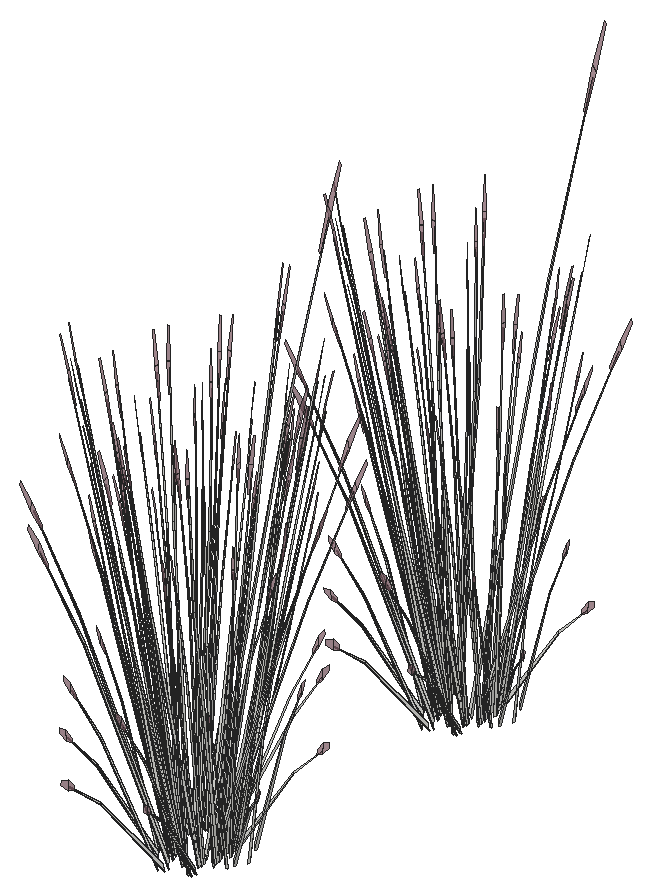
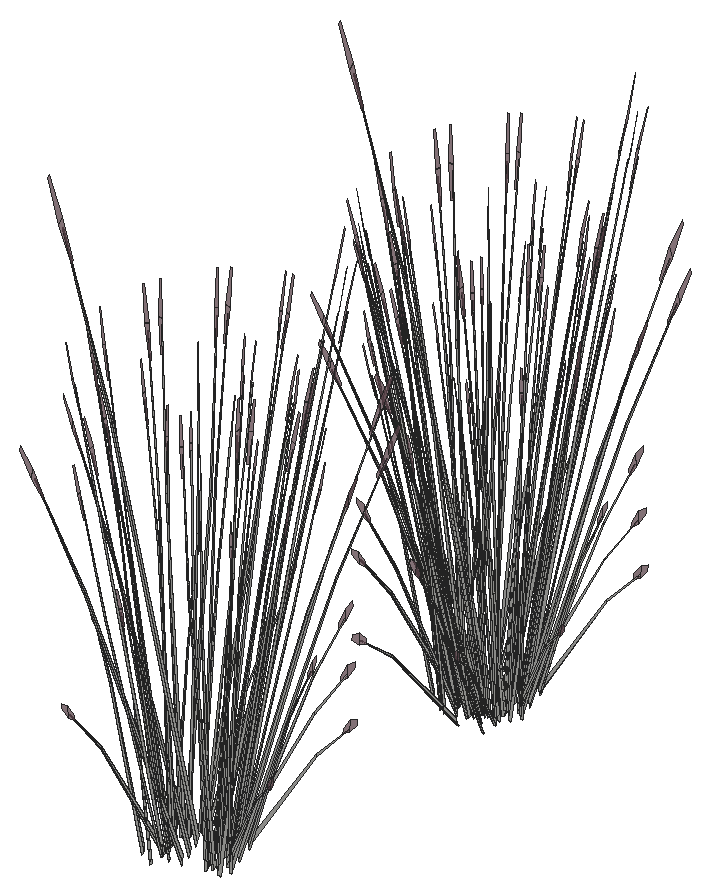
# SketchUp Ruby script. Lengths in inches.
U = 1.inch
M = Sketchup.active_model
def pt(a) = Geom::Point3d.new(a.map { |v| v * U })
def face(e, loops, mat)
  f = e.add_face(loops[0].map { |a| pt(a) })
  loops[1..].each { |l| e.add_face(l.map { |a| pt(a) }).erase! }
  f.material = f.back_material = mat if mat
  f
end
# faces: each face lists its corners as indices into pts; further lists are holes
def faces(e, pts, list, mat = nil) = list.each { |f| face(e, (f[0].is_a?(Array) ? f : [f]).map { |l| l.map { |i| pts[i] } }, mat) }
# xy, xz, yz: faces in a plane at the given z, y or x. An outline is a flat list of corners, or four numbers for a rectangle; further outlines are holes
def ring(l) = l.size == 4 ? [[l[0], l[1]], [l[2], l[1]], [l[2], l[3]], [l[0], l[3]]] : l.each_slice(2).to_a
def flat(e, list, mat, &to3) = list.each { |f| face(e, (f[0].is_a?(Array) ? f : [f]).map { |l| ring(l).map { |u, v| to3.(u, v) } }, mat) }
def xy(e, z, list, mat = nil) = flat(e, list, mat) { |x, y| [x, y, z] }
def xz(e, y, list, mat = nil) = flat(e, list, mat) { |x, z| [x, y, z] }
def yz(e, x, list, mat = nil) = flat(e, list, mat) { |y, z| [x, y, z] }
def lines(e, pts, list) = list.each { |a, b| e.add_line(pt(pts[a]), pt(pts[b])) }
# prism: a flat outline (further loops are holes) pulled along v
def prism(e, loops, v, mat = nil)
  f = face(e, loops, mat); d = Geom::Vector3d.new(v.map { |x| x * U })
  f.pushpull(f.normal.samedirection?(d) ? d.length : -d.length)
end
def box(e, o, s, mat = nil) = prism(e, [[o, [o[0] + s[0], o[1], o[2]], [o[0] + s[0], o[1] + s[1], o[2]], [o[0], o[1] + s[1], o[2]]]], [0, 0, s[2]], mat)
def at(x, y, z, deg = 0) = Geom::Transformation.translation(pt([x, y, z])) * Geom::Transformation.rotation(ORIGIN, Z_AXIS, deg.degrees)
def axes(o, x, y, z) = Geom::Transformation.new([*x, 0, *y, 0, *z, 0, *pt(o).to_a, 1])
def part(name) = M.definitions.add(name)
# library, detail: a bought-in or finely detailed component or shape, given as its bounding box
def library(name, o, s) = part(name).tap { |d| box(d.entities, o, s) }
def detail(e, o, s) = box(e.add_group.entities, o, s)
def put(e, d, t, mat = nil) = e.add_instance(d, t).tap { |i| i.material = mat if mat }
def group(e, t, mat = nil) = e.add_group.tap { |g| g.transformation = t; g.material = mat if mat }.entities
root = M.entities
M.materials.add("LightPink_Translucent").color = [144, 107, 117]
M.materials["LightPink_Translucent"].alpha = 0.75
c1 = part("blade")
p = [[2.15,0.21,22],[0,0.17,0],[0.09,0.45,0],[2.18,0.31,22],[2.29,0.31,22],[0.38,0.45,0],
  [2.48,0.24,33],[2.49,0.24,33],[2.48,0.22,33]]
faces(c1.entities,p,[[0,1,2,3],[4,5,2,3],[6,3,4,7],[8,0,3,6]])
c2 = part("seeds")
p = [[0.3,-0.1,1.38],[-0.01,-0.03,1.59],[-0.01,-0.03,0.03],[0.14,-0.07,-0.07],[0.29,-0.03,3],[0.15,0.01,3.11]]
faces(c2.entities,p,[[0,1,2,3],[1,0,4,5]],"LightPink_Translucent")
c3 = part("blade with seeds")
put(c3.entities,c1,at(0,0,0))
put(c3.entities,c2,axes([2.4,0.25,30.99],[1.5799,-0.05474,1.17369],[-0.12525,1.92788,0.29478],[-0.07173,-0.02425,1.56792]))
put(root,c3,axes([430.05,19.08,1.33],[0.08601,0.17716,1.47384],[-0.39746,0.14915,0.11917],[-0.08983,-0.27813,0.63005]))
put(root,c3,axes([430.7,17.9,2.05],[-0.05755,-0.07737,1.50452],[-0.38409,0.04905,-0.23794],[-0.0613,-0.18505,0.12066]))
put(root,c3,axes([432.43,18.85,2.05],[-0.00363,-0.10982,1.50452],[-0.30678,-0.3174,-0.23794],[0.04743,-0.1924,0.12066]))
put(root,c3,axes([431.39,19.39,1.33],[-0.07006,0.18966,1.47384],[-0.29392,-0.3925,0.11917],[0.13259,-0.24463,0.63005]))
put(root,c3,axes([432.35,18.46,2.05],[-0.03821,0.04215,1.5255],[-0.37441,-0.1422,-0.14414],[-0.01355,-0.18393,0.26996]))
put(root,c3,axes([430.31,17.65,2.05],[-0.00702,0.06614,1.5255],[-0.34622,0.24004,-0.14414],[-0.10188,-0.1227,0.26996]))
put(root,c3,axes([430.23,18.82,2.38],[0.41917,-0.14183,0.46236],[0.07275,0.55635,0.38124],[-0.09858,-0.16397,0.95674]))
put(root,c3,axes([431.18,18.93,2.07],[0.37078,0.14426,0.41282],[-0.12679,0.47426,0.34039],[-0.02228,-0.18651,0.85423]))
put(root,c3,axes([431.29,19.1,2.33],[-0.36822,0.25691,-0.10458],[-0.18095,-0.45596,-0.58045],[-0.04858,-0.19215,0.88199]))
put(root,c3,axes([432.05,19.67,2.33],[-0.41355,-0.02734,-0.10458],[0.0113,-0.51765,-0.58045],[0.02873,-0.19937,0.88199]))
put(root,c3,axes([431.28,18.89,2.07],[0.27727,-0.18753,0.0553],[0.13571,0.34197,0.43534],[-0.02678,-0.15075,0.66383]))
put(root,c3,axes([430.33,18.94,2.07],[0.17102,-0.35053,0.0553],[0.24354,0.20408,0.43534],[-0.07874,-0.11238,0.66383]))
put(root,c3,axes([429.47,19.63,1.33],[0.13977,0.09507,1.47384],[-0.28925,0.39884,0.11917],[-0.18028,-0.17992,0.63005]))
put(root,c3,axes([431.18,19.28,2.34],[-0.11344,0.42434,0.30456],[-0.33096,-0.12377,-0.39319],[-0.03035,-0.17085,0.75234]))
put(root,c3,axes([432.02,19.46,2.07],[0.26795,0.37649,0.41282],[-0.28456,0.3247,0.34039],[0.04943,-0.17664,0.85423]))
put(root,c3,axes([430.41,18.91,2.67],[-0.25113,0.52899,-0.11713],[-0.36369,-0.30476,-0.65011],[-0.12642,-0.14945,0.98783]))
put(root,c3,axes([432.12,19.49,2.07],[0.30922,0.02571,0.0553],[-0.00848,0.38824,0.43534],[0.03236,-0.14872,0.66383]))
put(root,c3,axes([431.89,19.75,2.34],[-0.2546,0.29052,0.30456],[-0.24101,-0.33173,-0.39319],[0.03667,-0.16855,0.75234]))
put(root,c3,axes([429.44,18.76,2.05],[-0.08096,-0.00389,1.50452],[-0.25776,0.38949,-0.23794],[-0.13753,-0.07958,0.12066]))
put(root,c3,axes([432.5,20.69,2.33],[-0.34807,-0.30426,-0.10458],[0.20053,-0.44063,-0.58045],[0.09834,-0.15317,0.88199]))
put(root,c3,axes([430.38,19.35,2.34],[0.05812,0.44446,0.30456],[-0.33222,0.11736,-0.39319],[-0.08923,-0.12737,0.75234]))
put(root,c3,axes([429.38,19.64,2.38],[0.31075,-0.40722,0.46236],[0.268,0.43246,0.38124],[-0.14579,-0.07512,0.95674]))
put(root,c3,axes([433.36,20.5625,2.05],[-0.04915,-0.00419,1.5255],[-0.20409,-0.44904,-0.14414],[0.08196,-0.14765,0.26996]))
put(root,c3,axes([429.53,19.63,2.07],[0.01895,-0.4196,0.0553],[0.28611,0.0115,0.43534],[-0.1096,-0.04391,0.66383]))
put(root,c3,axes([432.33,20.65,2.34],[-0.32754,0.07886,0.30456],[-0.08649,-0.45081,-0.39319],[0.09386,-0.12109,0.75234]))
put(root,c3,axes([432.63,20.58,2.07],[0.25832,0.23207,0.0553],[-0.1504,0.33047,0.43534],[0.08282,-0.10684,0.66383]))
put(root,c3,axes([432.56,20.48,2.07],[0.09332,0.50785,0.41282],[-0.36608,0.08814,0.34039],[0.10789,-0.11944,0.85423]))
put(root,c3,axes([433.54,21.1,2.05],[0.05222,-0.08405,1.50452],[-0.06683,-0.51557,-0.23794],[0.13101,-0.09775,0.12066]))
put(root,c3,axes([429.13,19.09,2.05],[0.0279,0.05507,1.5255],[-0.13448,0.49501,-0.14414],[-0.1362,0.00358,0.26996]))
put(root,c3,axes([429.72,19.95,2.34],[0.2141,0.34548,0.30456],[-0.24447,0.32704,-0.39319],[-0.12421,-0.04976,0.75234]))
put(root,c3,axes([429.66,19.73,2.33],[-0.02015,0.56117,-0.10458],[-0.38148,-0.01534,-0.58045],[-0.14692,-0.03898,0.88199]))
put(root,c3,axes([432.52,21.88,2.33],[-0.18933,-0.49965,-0.10458],[0.33602,-0.24554,-0.58045],[0.1416,-0.06592,0.88199]))
put(root,c3,axes([429.18,20.5,1.33],[0.15608,-0.0125,1.47384],[-0.10354,0.54165,0.11917],[-0.22242,-0.0335,0.63005]))
put(root,c3,axes([432.38,21.73,2.34],[-0.31272,-0.15393,0.30456],[0.09121,-0.44909,-0.39319],[0.1259,-0.04118,0.75234]))
put(root,c3,axes([429.11,20.91,2.07],[0.10631,-0.50312,0.41282],[0.34951,0.17204,0.34039],[-0.13745,0.03024,0.85423]))
put(root,c3,axes([429.08,20.78,2.07],[-0.1382,-0.37624,0.0553],[0.25202,-0.18416,0.43534],[-0.11109,0.03633,0.66383]))
put(root,c3,axes([431.86,21.125,1.33],[-0.15608,0.0125,1.47384],[0.10354,-0.54165,0.11917],[0.22242,0.0335,0.63005]))
put(root,c3,axes([432.67,21.87,2.07],[0.1382,0.37624,0.0553],[-0.25202,0.18416,0.43534],[0.11109,-0.03633,0.66383]))
put(root,c3,axes([432.64,21.74,2.07],[-0.10631,0.50312,0.41282],[-0.34951,-0.17204,0.34039],[0.13745,-0.03024,0.85423]))
put(root,c3,axes([429.37,20.92,2.34],[0.31272,0.15393,0.30456],[-0.09121,0.44909,-0.39319],[-0.1259,0.04118,0.75234]))
put(root,c3,axes([433.27,23.37,2.05],[-0.03403,-0.04831,1.5255],[0.07443,-0.51782,-0.14414],[0.13402,-0.03308,0.26996]))
put(root,c3,axes([428.84,21.26,2.05],[-0.06145,0.07164,1.50452],[0.00523,0.52344,-0.23794],[-0.14085,0.06807,0.12066]))
put(root,c3,axes([429.24,20.77,2.33],[0.18933,0.49965,-0.10458],[-0.33602,0.24554,-0.58045],[-0.1416,0.06592,0.88199]))
put(root,c3,axes([432.97,22.93,1.38],[-0.07202,-0.46385,-0.03003],[0.3404,-0.10664,-0.13615],[0.07108,0.02941,0.44908]))
put(root,c3,axes([432.09,22.92,2.33],[0.02015,-0.56117,-0.10458],[0.38148,0.01534,-0.58045],[0.14692,0.03898,0.88199]))
put(root,c3,axes([432.03,22.7,2.34],[-0.2141,-0.34548,0.30456],[0.24447,-0.32704,-0.39319],[0.12421,0.04976,0.75234]))
put(root,c3,axes([432.42,22.58,2.05],[0.08072,-0.00933,1.50452],[0.22141,-0.42869,-0.23794],[0.14358,0.05659,0.12066]))
put(root,c3,axes([429.2,22.16,2.07],[-0.09332,-0.50785,0.41282],[0.36608,-0.08814,0.34039],[-0.10789,0.11944,0.85423]))
put(root,c3,axes([429.125,22.07,2.07],[-0.25832,-0.23207,0.0553],[0.1504,-0.33047,0.43534],[-0.08282,0.10684,0.66383]))
put(root,c3,axes([429.24,21.45,1.33],[0.13056,-0.11672,1.47384],[0.10992,0.53933,0.11917],[-0.20497,0.12189,0.63005]))
put(root,c3,axes([429.42,21.99,2.34],[0.32754,-0.07886,0.30456],[0.08649,0.45081,-0.39319],[-0.09386,0.12109,0.75234]))
put(root,c3,axes([428.16,21.79,2.05],[0.04802,0.0148,1.5255],[0.14856,0.48754,-0.14414],[-0.0983,0.12796,0.26996]))
put(root,c3,axes([432.23,23.01,2.07],[-0.01895,0.4196,0.0553],[-0.28611,-0.0115,0.43534],[0.1096,0.04391,0.66383]))
put(root,c3,axes([432.25,22.88,2.07],[-0.27746,0.36359,0.41282],[-0.23929,-0.38612,0.34039],[0.13017,0.06707,0.85423]))
put(root,c3,axes([428.68,23.27,2.86],[0.33205,0.14729,-0.05579],[-0.10214,0.45334,-0.25298],[-0.05431,0.06883,0.83441]))
put(root,c3,axes([431.37,23.3,2.34],[-0.05812,-0.44446,0.30456],[0.33222,-0.11736,-0.39319],[0.08923,0.12737,0.75234]))
put(root,c3,axes([431.57,21.99,1.33],[-0.13977,-0.09507,1.47384],[0.28925,-0.39884,0.11917],[0.18028,0.17992,0.63005]))
put(root,c3,axes([431.59,20.74,1.85],[-0.32515,-0.2867,1.18923],[0.34333,-0.44639,0.51312],[0.10491,0.26901,1.1495]))
put(root,c3,axes([429.25,21.95,2.33],[0.34807,0.30426,-0.10458],[-0.20053,0.44063,-0.58045],[-0.09834,0.15317,0.88199]))
put(root,c3,axes([431.34,23.53,2.33],[0.22423,-0.47232,-0.10458],[0.32472,0.27211,-0.58045],[0.11288,0.13344,0.88199]))
put(root,c3,axes([429.72,21.82,1.33],[0.09398,-0.16955,1.47384],[0.23731,0.45764,0.11917],[-0.16276,0.20841,0.63005]))
put(root,c3,axes([429.86,22.89,2.34],[0.2546,-0.29052,0.30456],[0.24101,0.33173,-0.39319],[-0.03667,0.16855,0.75234]))
put(root,c3,axes([431.05,23.92,2.05],[0.00111,-0.06681,1.5255],[0.32247,-0.29474,-0.14414],[0.11201,0.1052,0.26996]))
put(root,c3,axes([429.63,23.16,2.07],[-0.30922,-0.02571,0.0553],[0.00848,-0.38824,0.43534],[-0.03236,0.14872,0.66383]))
put(root,c3,axes([429.73,23.19,2.07],[-0.26795,-0.37649,0.41282],[0.28456,-0.3247,0.34039],[-0.04943,0.17664,0.85423]))
put(root,c3,axes([430.58,23.37,2.34],[0.11344,-0.42434,0.30456],[0.33096,0.12377,-0.39319],[0.03035,0.17085,0.75234]))
put(root,c3,axes([431.42,23.7,2.07],[-0.17102,0.35053,0.0553],[-0.24354,-0.20408,0.43534],[0.07874,0.11238,0.66383]))
put(root,c3,axes([431.02,24.88,2.86],[0.26003,-0.31656,-0.05579],[0.23826,0.3467,-0.25298],[0.01677,0.09824,0.83441]))
put(root,c3,axes([431.5,23.6,2.07],[-0.37426,0.12663,0.41282],[-0.06495,-0.49674,0.34039],[0.08802,0.1464,0.85423]))
put(root,c3,axes([429.65,22.23,1.33],[0.07006,-0.18966,1.47384],[0.29392,0.3925,0.11917],[-0.13259,0.24463,0.63005]))
put(root,c3,axes([430.47,23.75,2.07],[-0.27727,0.18753,0.0553],[-0.13571,-0.34197,0.43534],[0.02678,0.15075,0.66383]))
put(root,c3,axes([428.85,23.22,2.05],[-0.00935,0.1092,1.50452],[0.26544,0.37987,-0.23794],[-0.06949,0.17964,0.12066]))
put(root,c3,axes([429.7,22.97,2.64],[0.41355,0.02734,-0.11608],[-0.0113,0.51765,-0.6443],[-0.02873,0.19937,0.97901]))
put(root,c3,axes([430.47,23.55,2.33],[0.36822,-0.25691,-0.10458],[0.18095,0.45596,-0.58045],[0.04858,0.19215,0.88199]))
put(root,c3,axes([430.57,23.72,2.35],[-0.37078,-0.14426,0.45823],[0.12679,-0.47426,0.37783],[0.02228,0.18651,0.9482]))
put(root,c3,axes([430.99,22.55,1.33],[-0.08601,-0.17716,1.47384],[0.39746,-0.14915,0.11917],[0.08983,0.27813,0.63005]))
put(root,c3,axes([428.82,24.34,2.05],[0.04269,-0.03331,1.5255],[0.35284,0.2216,-0.14414],[-0.00829,0.1845,0.26996]))
put(root,c3,axes([430.29,22.63,1.33],[-0.00921,-0.21179,1.47384],[0.39917,0.1405,0.11917],[-0.02469,0.30182,0.63005]))
put(root,c3,axes([430.38,24.57,2.05],[0.0477,0.08886,1.50452],[0.38493,0.03491,-0.23794],[0.03871,0.19596,0.12066]))
put(root,c3,axes([431.68,42.12,1.33],[0.08601,0.17716,1.47384],[-0.39746,0.14915,0.11917],[-0.08983,-0.27813,0.63005]))
put(root,c3,axes([432.33,40.95,2.05],[-0.05755,-0.07737,1.50452],[-0.38409,0.04905,-0.23794],[-0.0613,-0.18505,0.12066]))
put(root,c3,axes([434.06,41.89,2.05],[-0.00363,-0.10982,1.50452],[-0.30678,-0.3174,-0.23794],[0.04743,-0.1924,0.12066]))
put(root,c3,axes([433.02,42.43,1.33],[-0.07006,0.18966,1.47384],[-0.29392,-0.3925,0.11917],[0.13259,-0.24463,0.63005]))
put(root,c3,axes([433.98,41.5,2.05],[-0.03821,0.04215,1.5255],[-0.37441,-0.1422,-0.14414],[-0.01355,-0.18393,0.26996]))
put(root,c3,axes([431.9375,40.69,2.05],[-0.00702,0.06614,1.5255],[-0.34622,0.24004,-0.14414],[-0.10188,-0.1227,0.26996]))
put(root,c3,axes([431.86,41.87,2.38],[0.41917,-0.14183,0.46236],[0.07275,0.55635,0.38124],[-0.09858,-0.16397,0.95674]))
put(root,c3,axes([432.81,41.97,2.07],[0.37078,0.14426,0.41282],[-0.12679,0.47426,0.34039],[-0.02228,-0.18651,0.85423]))
put(root,c3,axes([432.92,42.14,2.33],[-0.36822,0.25691,-0.10458],[-0.18095,-0.45596,-0.58045],[-0.04858,-0.19215,0.88199]))
put(root,c3,axes([433.68,42.72,2.33],[-0.41355,-0.02734,-0.10458],[0.0113,-0.51765,-0.58045],[0.02873,-0.19937,0.88199]))
put(root,c3,axes([432.91,41.93,2.07],[0.27727,-0.18753,0.0553],[0.13571,0.34197,0.43534],[-0.02678,-0.15075,0.66383]))
put(root,c3,axes([431.96,41.99,2.07],[0.17102,-0.35053,0.0553],[0.24354,0.20408,0.43534],[-0.07874,-0.11238,0.66383]))
put(root,c3,axes([431.1,42.67,1.33],[0.13977,0.09507,1.47384],[-0.28925,0.39884,0.11917],[-0.18028,-0.17992,0.63005]))
put(root,c3,axes([432.81,42.32,2.34],[-0.11344,0.42434,0.30456],[-0.33096,-0.12377,-0.39319],[-0.03035,-0.17085,0.75234]))
put(root,c3,axes([433.65,42.5,2.07],[0.26795,0.37649,0.41282],[-0.28456,0.3247,0.34039],[0.04943,-0.17664,0.85423]))
put(root,c3,axes([432.04,41.95,2.67],[-0.25113,0.52899,-0.11713],[-0.36369,-0.30476,-0.65011],[-0.12642,-0.14945,0.98783]))
put(root,c3,axes([433.75,42.53,2.07],[0.30922,0.02571,0.0553],[-0.00848,0.38824,0.43534],[0.03236,-0.14872,0.66383]))
put(root,c3,axes([433.52,42.8,2.34],[-0.2546,0.29052,0.30456],[-0.24101,-0.33173,-0.39319],[0.03667,-0.16855,0.75234]))
put(root,c3,axes([431.07,41.8,2.05],[-0.08096,-0.00389,1.50452],[-0.25776,0.38949,-0.23794],[-0.13753,-0.07958,0.12066]))
put(root,c3,axes([434.13,43.73,2.33],[-0.34807,-0.30426,-0.10458],[0.20053,-0.44063,-0.58045],[0.09834,-0.15317,0.88199]))
put(root,c3,axes([432.01,42.39,2.34],[0.05812,0.44446,0.30456],[-0.33222,0.11736,-0.39319],[-0.08923,-0.12737,0.75234]))
put(root,c3,axes([431.01,42.68,2.38],[0.31075,-0.40722,0.46236],[0.268,0.43246,0.38124],[-0.14579,-0.07512,0.95674]))
put(root,c3,axes([434.99,43.6,2.05],[-0.04915,-0.00419,1.5255],[-0.20409,-0.44904,-0.14414],[0.08196,-0.14765,0.26996]))
put(root,c3,axes([431.16,42.68,2.07],[0.01895,-0.4196,0.0553],[0.28611,0.0115,0.43534],[-0.1096,-0.04391,0.66383]))
put(root,c3,axes([433.96,43.69,2.34],[-0.32754,0.07886,0.30456],[-0.08649,-0.45081,-0.39319],[0.09386,-0.12109,0.75234]))
put(root,c3,axes([434.26,43.62,2.07],[0.25832,0.23207,0.0553],[-0.1504,0.33047,0.43534],[0.08282,-0.10684,0.66383]))
put(root,c3,axes([434.1875,43.52,2.07],[0.09332,0.50785,0.41282],[-0.36608,0.08814,0.34039],[0.10789,-0.11944,0.85423]))
put(root,c3,axes([435.17,44.14,2.05],[0.05222,-0.08405,1.50452],[-0.06683,-0.51557,-0.23794],[0.13101,-0.09775,0.12066]))
put(root,c3,axes([430.76,42.13,2.05],[0.0279,0.05507,1.5255],[-0.13448,0.49501,-0.14414],[-0.1362,0.00358,0.26996]))
put(root,c3,axes([431.35,42.99,2.34],[0.2141,0.34548,0.30456],[-0.24447,0.32704,-0.39319],[-0.12421,-0.04976,0.75234]))
put(root,c3,axes([431.29,42.77,2.33],[-0.02015,0.56117,-0.10458],[-0.38148,-0.01534,-0.58045],[-0.14692,-0.03898,0.88199]))
put(root,c3,axes([434.15,44.92,2.33],[-0.18933,-0.49965,-0.10458],[0.33602,-0.24554,-0.58045],[0.1416,-0.06592,0.88199]))
put(root,c3,axes([430.81,43.54,1.33],[0.15608,-0.0125,1.47384],[-0.10354,0.54165,0.11917],[-0.22242,-0.0335,0.63005]))
put(root,c3,axes([434.01,44.77,2.34],[-0.31272,-0.15393,0.30456],[0.09121,-0.44909,-0.39319],[0.1259,-0.04118,0.75234]))
put(root,c3,axes([430.74,43.95,2.07],[0.10631,-0.50312,0.41282],[0.34951,0.17204,0.34039],[-0.13745,0.03024,0.85423]))
put(root,c3,axes([430.71,43.82,2.07],[-0.1382,-0.37624,0.0553],[0.25202,-0.18416,0.43534],[-0.11109,0.03633,0.66383]))
put(root,c3,axes([433.49,44.17,1.33],[-0.15608,0.0125,1.47384],[0.10354,-0.54165,0.11917],[0.22242,0.0335,0.63005]))
put(root,c3,axes([434.3,44.91,2.07],[0.1382,0.37624,0.0553],[-0.25202,0.18416,0.43534],[0.11109,-0.03633,0.66383]))
put(root,c3,axes([434.27,44.78,2.07],[-0.10631,0.50312,0.41282],[-0.34951,-0.17204,0.34039],[0.13745,-0.03024,0.85423]))
put(root,c3,axes([431,43.96,2.34],[0.31272,0.15393,0.30456],[-0.09121,0.44909,-0.39319],[-0.1259,0.04118,0.75234]))
put(root,c3,axes([434.9,46.41,2.05],[-0.03403,-0.04831,1.5255],[0.07443,-0.51782,-0.14414],[0.13402,-0.03308,0.26996]))
put(root,c3,axes([430.47,44.31,2.05],[-0.06145,0.07164,1.50452],[0.00523,0.52344,-0.23794],[-0.14085,0.06807,0.12066]))
put(root,c3,axes([430.87,43.81,2.33],[0.18933,0.49965,-0.10458],[-0.33602,0.24554,-0.58045],[-0.1416,0.06592,0.88199]))
put(root,c3,axes([434.6,45.97,1.38],[-0.07202,-0.46385,-0.03003],[0.3404,-0.10664,-0.13615],[0.07108,0.02941,0.44908]))
put(root,c3,axes([433.72,45.96,2.33],[0.02015,-0.56117,-0.10458],[0.38148,0.01534,-0.58045],[0.14692,0.03898,0.88199]))
put(root,c3,axes([433.66,45.74,2.34],[-0.2141,-0.34548,0.30456],[0.24447,-0.32704,-0.39319],[0.12421,0.04976,0.75234]))
put(root,c3,axes([434.05,45.625,2.05],[0.08072,-0.00933,1.50452],[0.22141,-0.42869,-0.23794],[0.14358,0.05659,0.12066]))
put(root,c3,axes([430.82,45.2,2.07],[-0.09332,-0.50785,0.41282],[0.36608,-0.08814,0.34039],[-0.10789,0.11944,0.85423]))
put(root,c3,axes([430.75,45.11,2.07],[-0.25832,-0.23207,0.0553],[0.1504,-0.33047,0.43534],[-0.08282,0.10684,0.66383]))
put(root,c3,axes([430.87,44.49,1.33],[0.13056,-0.11672,1.47384],[0.10992,0.53933,0.11917],[-0.20497,0.12189,0.63005]))
put(root,c3,axes([431.05,45.04,2.34],[0.32754,-0.07886,0.30456],[0.08649,0.45081,-0.39319],[-0.09386,0.12109,0.75234]))
put(root,c3,axes([429.79,44.83,2.05],[0.04802,0.0148,1.5255],[0.14856,0.48754,-0.14414],[-0.0983,0.12796,0.26996]))
put(root,c3,axes([433.86,46.05,2.07],[-0.01895,0.4196,0.0553],[-0.28611,-0.0115,0.43534],[0.1096,0.04391,0.66383]))
put(root,c3,axes([433.88,45.92,2.07],[-0.27746,0.36359,0.41282],[-0.23929,-0.38612,0.34039],[0.13017,0.06707,0.85423]))
put(root,c3,axes([430.31,46.32,2.86],[0.33205,0.14729,-0.05579],[-0.10214,0.45334,-0.25298],[-0.05431,0.06883,0.83441]))
put(root,c3,axes([433,46.34,2.34],[-0.05812,-0.44446,0.30456],[0.33222,-0.11736,-0.39319],[0.08923,0.12737,0.75234]))
put(root,c3,axes([433.2,45.04,1.33],[-0.13977,-0.09507,1.47384],[0.28925,-0.39884,0.11917],[0.18028,0.17992,0.63005]))
put(root,c3,axes([433.22,43.78,1.85],[-0.32515,-0.2867,1.18923],[0.34333,-0.44639,0.51312],[0.10491,0.26901,1.1495]))
put(root,c3,axes([430.88,44.99,2.33],[0.34807,0.30426,-0.10458],[-0.20053,0.44063,-0.58045],[-0.09834,0.15317,0.88199]))
